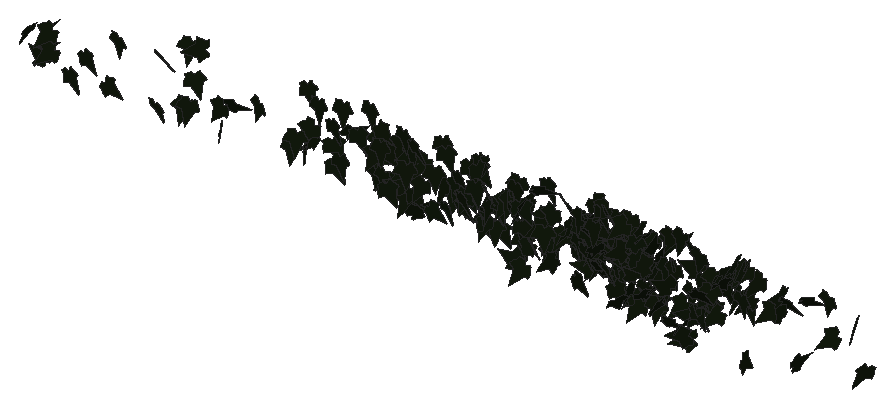
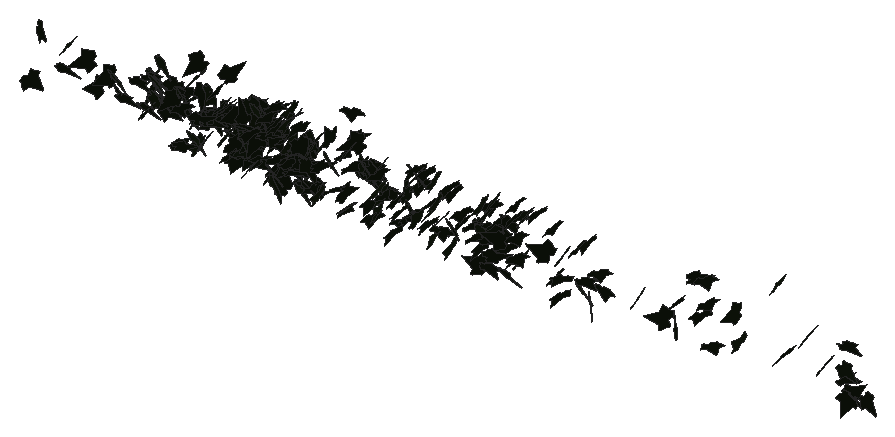
# SketchUp Ruby script. Lengths in inches.
U = 1.inch
M = Sketchup.active_model
def pt(a) = Geom::Point3d.new(a.map { |v| v * U })
def face(e, loops, mat)
  f = e.add_face(loops[0].map { |a| pt(a) })
  loops[1..].each { |l| e.add_face(l.map { |a| pt(a) }).erase! }
  f.material = f.back_material = mat if mat
  f
end
# faces: each face lists its corners as indices into pts; further lists are holes
def faces(e, pts, list, mat = nil) = list.each { |f| face(e, (f[0].is_a?(Array) ? f : [f]).map { |l| l.map { |i| pts[i] } }, mat) }
# xy, xz, yz: faces in a plane at the given z, y or x. An outline is a flat list of corners, or four numbers for a rectangle; further outlines are holes
def ring(l) = l.size == 4 ? [[l[0], l[1]], [l[2], l[1]], [l[2], l[3]], [l[0], l[3]]] : l.each_slice(2).to_a
def flat(e, list, mat, &to3) = list.each { |f| face(e, (f[0].is_a?(Array) ? f : [f]).map { |l| ring(l).map { |u, v| to3.(u, v) } }, mat) }
def xy(e, z, list, mat = nil) = flat(e, list, mat) { |x, y| [x, y, z] }
def xz(e, y, list, mat = nil) = flat(e, list, mat) { |x, z| [x, y, z] }
def yz(e, x, list, mat = nil) = flat(e, list, mat) { |y, z| [x, y, z] }
def lines(e, pts, list) = list.each { |a, b| e.add_line(pt(pts[a]), pt(pts[b])) }
# prism: a flat outline (further loops are holes) pulled along v
def prism(e, loops, v, mat = nil)
  f = face(e, loops, mat); d = Geom::Vector3d.new(v.map { |x| x * U })
  f.pushpull(f.normal.samedirection?(d) ? d.length : -d.length)
end
def box(e, o, s, mat = nil) = prism(e, [[o, [o[0] + s[0], o[1], o[2]], [o[0] + s[0], o[1] + s[1], o[2]], [o[0], o[1] + s[1], o[2]]]], [0, 0, s[2]], mat)
def at(x, y, z, deg = 0) = Geom::Transformation.translation(pt([x, y, z])) * Geom::Transformation.rotation(ORIGIN, Z_AXIS, deg.degrees)
def axes(o, x, y, z) = Geom::Transformation.new([*x, 0, *y, 0, *z, 0, *pt(o).to_a, 1])
def part(name) = M.definitions.add(name)
# library, detail: a bought-in or finely detailed component or shape, given as its bounding box
def library(name, o, s) = part(name).tap { |d| box(d.entities, o, s) }
def detail(e, o, s) = box(e.add_group.entities, o, s)
def put(e, d, t, mat = nil) = e.add_instance(d, t).tap { |i| i.material = mat if mat }
def group(e, t, mat = nil) = e.add_group.tap { |g| g.transformation = t; g.material = mat if mat }.entities
root = M.entities
M.materials.add("efeu1").color = [18, 25, 13]
c1 = part("ivyleaf_9")
p = [[1.54,2.16,1.25],[1.36,2.04,1.19],[-0.21,0.99,0.68],[-0.71,1.11,0.82],[-0.85,0.86,0.67],[-0.8,0.17,0.21],
  [-0.9,-0.01,0.1],[-0.67,-0.16,-0.02],[-0.08,-0.08,-0.05],[-0.03,-0.6,-0.4],[0.65,-0.88,-0.66],[0.83,-0.6,-0.49],
  [1.29,-0.42,-0.43],[1.8125,-0.07,-0.26],[1.21,0.44,0.15]]
faces(c1.entities,p,[[0,1,2,3,4,5,6,7,8,9,10,11,12,13,14]],"efeu1")
put(root,c1,axes([46.6,216.37,258.25],[-0.27202,-0.34629,-0.23682],[0.19921,0.14178,-0.43614],[0.36922,-0.33163,0.06083]))
put(root,c1,axes([55.82,216.69,257.36],[0.0222,0.00311,0.4995],[-0.43747,-0.24121,0.02095],[0.2411,-0.43796,-0.00798]))
put(root,c1,axes([44.75,216.71,254.99],[-0.44174,-0.23377,0.01468],[-0.01267,-0.00744,-0.49978],[0.23389,-0.44192,0.00065]))
put(root,c1,axes([51.99,216.38,255.35],[0.13956,0.47976,-0.01875],[-0.00594,-0.0178,-0.49965],[-0.48009,0.13969,0.00073]))
put(root,c1,axes([57.05,216.84,254.52],[-0.16748,-0.06607,-0.46646],[-0.30465,-0.36244,0.16072],[-0.35936,0.33804,0.08114]))
put(root,c1,axes([57.76,216.6,257.77],[0.46943,0.14872,0.08669],[0.08408,0.02166,-0.4924],[-0.15022,0.47688,-0.00467]))
put(root,c1,axes([50.58,216.97,257.02],[0.32423,-0.35893,0.12668],[0.07945,-0.09892,-0.48364],[0.37224,0.33374,-0.00711]))
put(root,c1,axes([61.5,216.62,254.54],[0.14205,-0.0765,-0.47325],[-0.35114,0.31944,-0.15703],[0.32638,0.37697,0.03702]))
put(root,c1,axes([57.02,217.34,253.99],[-0.31084,-0.10965,0.37597],[-0.32126,-0.20314,-0.32485],[0.22399,-0.44352,0.05583]))
put(root,c1,axes([56.46,217.125,254.9],[-0.19577,0.41436,-0.19996],[0.08916,-0.17901,-0.45826],[-0.45136,-0.21508,-0.0038]))
put(root,c1,axes([55.3125,216.99,254.87],[0.44843,-0.00718,0.22104],[0.22112,0.02369,-0.44782],[-0.00405,0.49939,0.02442]))
put(root,c1,axes([45.39,217.83,257.31],[-0.21869,-0.24197,0.37898],[-0.22849,-0.30316,-0.3254],[0.38726,-0.31551,0.02202]))
put(root,c1,axes([43.55,217.49,254.54],[-0.15058,0.15267,0.45168],[-0.42718,0.16718,-0.19892],[-0.21176,-0.4458,0.08009]))
put(root,c1,axes([12.92,217.94,258.77],[0.08923,-0.44015,0.21978],[0.07683,-0.20816,-0.44807],[0.48594,0.11373,0.03048]))
put(root,c1,axes([44.5,217.96,255.54],[-0.00907,-0.19475,0.46042],[0.18666,-0.42852,-0.17758],[0.46376,0.16867,0.08047]))
put(root,c1,axes([50.88,217.7,255.39],[0.15521,-0.37076,-0.2974],[-0.03273,0.30378,-0.39579],[0.47417,0.14233,0.07003]))
put(root,c1,axes([56.61,218.16,255.05],[-0.21741,0.01252,0.45009],[-0.3715,-0.28738,-0.17145],[0.2544,-0.40897,0.13426]))
put(root,c1,axes([51.73,218.16,255.46],[-0.16544,0.16469,-0.44216],[0.31866,-0.30655,-0.23341],[-0.34797,-0.35903,-0.00352]))
put(root,c1,axes([53.93,217.61,254.95],[0.08311,0.39802,0.29098],[0.07803,0.28075,-0.40631],[-0.48683,0.11295,-0.01545]))
put(root,c1,axes([51.03,218.4,257.45],[-0.17348,-0.17204,0.43624],[-0.29823,-0.31848,-0.24419],[0.36189,-0.34492,0.00789]))
put(root,c1,axes([52.95,218.23,257.14],[-0.34233,0.00365,0.36441],[-0.36442,0.00068,-0.34234],[-0.00299,-0.49999,0.0022]))
put(root,c1,axes([44,218.26,255.5],[-0.49518,-0.06094,-0.03293],[0.0327,0.00393,-0.49891],[0.06106,-0.49626,0.00009]))
put(root,c1,axes([55.6875,218.3,255.66],[-0.48249,-0.12906,0.02348],[-0.02308,-0.00461,-0.49945],[0.12913,-0.48303,-0.00151]))
put(root,c1,axes([8.98,218.17,255],[0.23883,-0.4254,-0.10953],[-0.03464,0.10604,-0.4874],[0.43791,0.2404,0.02117]))
put(root,c1,axes([18,218.39,256],[-0.17042,-0.46998,-0.00871],[-0.00292,0.01032,-0.49988],[0.47005,-0.17033,-0.00627]))
put(root,c1,axes([38.69,218.25,257.01],[0.3155,-0.38699,0.02646],[0.01015,-0.02586,-0.49923],[0.38776,0.31555,-0.00846]))
put(root,c1,axes([10.19,218.15,256.64],[0.27225,-0.38072,-0.17588],[-0.05784,0.1736,-0.46531],[0.41537,0.27371,0.05048]))
put(root,c1,axes([52.14,218.26,257.62],[0.07993,-0.37701,-0.31856],[-0.0011,0.32257,-0.38203],[0.49357,0.06177,0.05074]))
put(root,c1,axes([7.3,218.61,257.05],[-0.45431,-0.19542,0.07356],[-0.07134,-0.02028,-0.49447],[0.19624,-0.45978,-0.00946]))
put(root,c1,axes([56.44,218.5,255.39],[0.18945,-0.43156,-0.16691],[-0.06005,0.15591,-0.47126],[0.45881,0.19861,0.00725]))
put(root,c1,axes([51.76,218.54,255.93],[0.06218,0.09947,0.48604],[-0.49051,0.08578,0.0452],[-0.07439,-0.48244,0.10825]))
put(root,c1,axes([64.18,218.15,254.37],[0.07503,0.11513,0.48074],[0.29064,0.38305,-0.1371],[-0.39987,0.30002,-0.00944]))
put(root,c1,axes([34.2,218.72,257.2],[-0.16152,-0.45144,-0.14182],[0.04335,0.13511,-0.47944],[0.4712,-0.16717,-0.0045]))
put(root,c1,axes([36.31,218.41,255.3],[0.2751,-0.28143,-0.3084],[-0.09944,0.31454,-0.37574],[0.4055,0.26807,0.11709]))
put(root,c1,axes([31.8,218.94,257.28],[-0.20715,-0.42551,0.16133],[-0.03674,-0.16104,-0.47193],[0.45359,-0.20737,0.03545]))
put(root,c1,axes([32.16,218.84,257.95],[0.01535,-0.49936,0.02005],[0.00157,-0.02001,-0.4996],[0.49976,0.0154,0.00095]))
put(root,c1,axes([11.61,218.45,255.0625],[0.28954,-0.28549,-0.29097],[-0.07063,0.31636,-0.38069],[0.40147,0.26155,0.14287]))
put(root,c1,axes([59.54,218.91,257.1],[0.1146,-0.46397,0.14697],[0.06046,-0.13625,-0.47726],[0.48292,0.12716,0.02488]))
put(root,c1,axes([51.8,218.98,253.98],[-0.35344,-0.34688,0.06897],[-0.0423,-0.05534,-0.49512],[0.35113,-0.35583,0.00977]))
put(root,c1,axes([48.54,218.79,255.3],[0.24621,-0.18445,0.39415],[0.33599,-0.20724,-0.30686],[0.27657,0.41597,0.0219]))
put(root,c1,axes([51.61,218.85,258.23],[-0.29685,-0.24752,-0.3172],[0.30386,0.12045,-0.37836],[0.26372,-0.4174,0.07891]))
put(root,c1,axes([57.3,218.85,256.98],[-0.29515,-0.33546,-0.22439],[0.16685,0.15171,-0.44626],[0.36749,-0.33831,0.02238]))
put(root,c1,axes([57,219.11,256.3],[-0.2397,-0.33909,0.2785],[-0.02799,-0.30488,-0.3953],[0.43791,-0.2051,0.12717]))
put(root,c1,axes([14.9375,218.95,254.57],[0.20312,-0.40476,0.21192],[0.14685,-0.16178,-0.44974],[0.43264,0.24494,0.05315]))
put(root,c1,axes([46.95,218.88,254.0625],[-0.00252,-0.04185,-0.49824],[0.4782,0.14529,-0.01462],[0.146,-0.47659,0.0393]))
put(root,c1,axes([44.99,219.23,254.45],[0.00054,-0.18494,-0.46454],[0.18893,-0.43002,0.17142],[-0.46293,-0.17572,0.06942]))
put(root,c1,axes([30.33,218.94,258.12],[0.10182,-0.46175,-0.16255],[0.03884,0.17312,-0.46746],[0.48798,0.08256,0.07112]))
put(root,c1,axes([46.87,219.21,256.47],[0.13455,-0.44972,0.17217],[0.05309,-0.16382,-0.46941],[0.47862,0.1446,0.00366]))
put(root,c1,axes([51.33,218.93,254.42],[0.02387,-0.38738,-0.31522],[0.11928,0.31087,-0.373],[0.48498,-0.05739,0.10725]))
put(root,c1,axes([48.82,219.1,255.74],[-0.4367,0.13125,-0.2051],[0.18228,-0.10302,-0.45405],[-0.16145,-0.47134,0.04213]))
put(root,c1,axes([53.73,219.13,257.28],[-0.37507,-0.11711,-0.3092],[0.29288,0.09933,-0.39288],[0.15345,-0.47584,-0.00592]))
put(root,c1,axes([52.93,219.24,254.33],[-0.14871,-0.47622,-0.03324],[0.00979,0.03176,-0.49889],[0.47727,-0.14903,-0.00012]))
put(root,c1,axes([50.2,219.23,257.27],[0.0615,-0.49608,0.01088],[-0.00534,-0.01163,-0.49984],[0.49617,0.06136,-0.00673]))
put(root,c1,axes([54.16,219.37,257.08],[-0.03919,-0.46359,0.18317],[0.0017,-0.18386,-0.46497],[0.49846,-0.03582,0.01599]))
put(root,c1,axes([32.47,219.05,255.14],[0.07068,-0.42142,-0.25964],[0.01915,0.26441,-0.42394],[0.49461,0.04999,0.05352]))
put(root,c1,axes([6.82,219.39,255.21],[-0.3187,-0.30322,0.23768],[-0.17883,-0.15679,-0.43981],[0.34125,-0.36534,-0.00851]))
put(root,c1,axes([38.01,219.03,255.89],[0.34804,-0.30238,-0.19348],[-0.09375,0.18356,-0.45554],[0.34652,0.35337,0.07108]))
put(root,c1,axes([51.11,219.29,256.08],[-0.23991,0.03835,0.437],[-0.43764,-0.05521,-0.23542],[0.0302,-0.49546,0.06006]))
put(root,c1,axes([19.54,219.53,255.84],[-0.13919,-0.38832,0.28255],[-0.02579,-0.28771,-0.40812],[0.47954,-0.12818,0.06006]))
put(root,c1,axes([51.93,218.82,254.7],[0.27637,0.4073,0.08789],[0.04051,0.0787,-0.4921],[-0.4147,0.27912,0.0105]))
put(root,c1,axes([50.17,219.55,258.52],[-0.28732,-0.33465,0.2355],[-0.12388,-0.20312,-0.43977],[0.39,-0.31105,0.03381]))
put(root,c1,axes([55.93,219.54,258.43],[-0.02564,-0.44129,0.23367],[0.07628,-0.2347,-0.43486],[0.49348,0.01335,0.07936]))
put(root,c1,axes([38.08,219.5625,256.24],[-0.14057,-0.44203,0.18669],[0.02208,-0.20028,-0.4576],[0.47933,-0.1204,0.07582]))
put(root,c1,axes([25.34,219.4,255.98],[-0.23511,-0.41805,-0.14128],[0.11602,0.09588,-0.47681],[0.42575,-0.25699,0.05191]))
put(root,c1,axes([47.24,219.42,255.93],[0.19824,-0.44635,0.10709],[0.04649,-0.09653,-0.48839],[0.45666,0.20359,0.00323]))
put(root,c1,axes([6.26,219.26,254.35],[0.05843,0.08654,0.43977],[-0.46088,0.07463,0.0409],[-0.0699,-0.41972,0.09794]))
put(root,c1,axes([19.44,219.41,253.81],[-0.0579,0.27116,0.41608],[0.00919,-0.41824,0.27385],[0.49655,0.03937,0.04345]))
put(root,c1,axes([51.8,219.36,258.32],[-0.25272,0.35464,-0.24569],[0.01565,-0.27701,-0.41595],[-0.43115,-0.21793,0.12892]))
put(root,c1,axes([42.44,219.27,257.32],[-0.11561,-0.25294,-0.41552],[0.26195,0.32751,-0.27225],[0.4099,-0.28064,0.05679]))
put(root,c1,axes([50.92,219.54,256.4],[-0.42153,-0.11595,-0.24263],[0.25964,-0.05806,-0.42334],[0.07,-0.48289,0.10916]))
put(root,c1,axes([57.39,219.28,257],[-0.37985,0.32233,0.04262],[-0.03893,0.01998,-0.49808],[-0.3228,-0.38171,0.00992]))
put(root,c1,axes([38.875,219.47,257.24],[-0.01632,-0.48334,-0.12694],[-0.00554,0.12718,-0.48352],[0.4997,-0.01437,-0.00951]))
put(root,c1,axes([57.7,219.07,257.33],[0.1816,0.46233,0.05721],[0.029,0.05007,-0.49664],[-0.46495,0.18369,-0.00863]))
put(root,c1,axes([58.875,219.55,256.9],[-0.4172,0.05536,-0.26996],[0.26086,-0.07858,-0.41926],[-0.08885,-0.49067,0.03668]))
put(root,c1,axes([48.04,219.52,256.23],[-0.08518,0.30537,-0.38664],[0.08176,-0.37818,-0.3167],[-0.48586,-0.11718,0.01449]))
put(root,c1,axes([44.61,219.75,257.34],[-0.14301,-0.44657,0.17356],[-0.03051,-0.17227,-0.46839],[0.47814,-0.14456,0.02203]))
put(root,c1,axes([39.48,219.71,255.04],[-0.14928,-0.46948,0.08546],[-0.0198,-0.08338,-0.4926],[0.47678,-0.15045,0.0063]))
put(root,c1,axes([42.54,219.63,257.2],[-0.20433,0.20114,-0.40962],[0.19872,-0.36481,-0.27826],[-0.41081,-0.27651,0.06914]))
put(root,c1,axes([24.83,219.67,255.18],[-0.36365,-0.22218,-0.26152],[0.24509,0.09856,-0.42452],[0.24019,-0.43694,0.03723]))
put(root,c1,axes([43.96,219.85,256.8125],[-0.19323,-0.44485,0.12152],[-0.03486,-0.11729,-0.4848],[0.45983,-0.19583,0.01431]))
put(root,c1,axes([58.67,219.51,258.83],[-0.35517,0.34586,-0.06512],[0.04753,-0.04453,-0.49574],[-0.34871,-0.35833,-0.00124]))
put(root,c1,axes([47.68,219.8,257.49],[-0.01573,-0.4963,0.05865],[-0.00361,-0.05856,-0.49655],[0.49974,-0.01605,-0.00174]))
put(root,c1,axes([67.64,219.72,257.95],[-0.24893,0.16868,-0.39947],[0.34126,-0.20799,-0.30048],[-0.26754,-0.42224,-0.01157]))
put(root,c1,axes([31.91,219.58,257.21],[-0.04556,-0.19176,-0.45952],[0.40278,0.25709,-0.14722],[0.29274,-0.38358,0.13105]))
put(root,c1,axes([47.2,219.74,256.875],[0.09362,-0.49074,-0.02032],[-0.00635,0.01947,-0.49958],[0.49112,0.0938,-0.00259]))
put(root,c1,axes([51.35,219.27,256.04],[0.39024,0.27499,0.14864],[0.12242,0.08432,-0.47739],[-0.28763,0.40898,-0.00152]))
put(root,c1,axes([49.41,219.95,254.32],[-0.06597,-0.38801,0.30838],[0.08309,-0.31536,-0.37901],[0.48862,0.00124,0.10608]))
put(root,c1,axes([46.54,219.96,257.63],[-0.03361,-0.4324,0.24879],[0.01186,-0.24998,-0.43286],[0.49873,-0.0232,0.02706]))
put(root,c1,axes([45.82,219.69,256.78],[-0.43317,0.19042,-0.16156],[0.14963,-0.06106,-0.47316],[-0.19993,-0.45827,-0.00409]))
put(root,c1,axes([46.97,219.52,256.74],[0.34698,-0.06127,0.35475],[0.35388,-0.03248,-0.35173],[0.06615,0.49517,0.02082]))
put(root,c1,axes([48.15,219.74,258.73],[0.21227,-0.45054,-0.04421],[-0.01463,0.04198,-0.49802],[0.45247,0.21273,0.00464]))
put(root,c1,axes([38.26,219.67,258.42],[0.05787,-0.45014,-0.20982],[-0.02566,0.20825,-0.45384],[0.49598,0.06329,0.00101]))
put(root,c1,axes([39.46,219.65,255],[0.11746,-0.43417,-0.2184],[0.01219,0.22724,-0.44521],[0.48585,0.09927,0.06397]))
put(root,c1,axes([45.36,219.93,258.125],[0.04871,-0.28251,0.40965],[0.23061,-0.35193,-0.27012],[0.44096,0.21525,0.09601]))
put(root,c1,axes([55.43,219.78,254.25],[0.32276,-0.34337,0.16709],[0.12139,-0.11518,-0.47117],[0.36206,0.34472,0.00901]))
put(root,c1,axes([38.92,219.62,258.45],[0.1207,-0.39132,-0.28688],[0.02892,0.3009,-0.39828],[0.48435,0.07955,0.09527]))
put(root,c1,axes([30.82,220,255.07],[0.06163,-0.43045,0.24682],[0.07195,-0.23833,-0.43361],[0.49094,0.08896,0.03257]))
put(root,c1,axes([51.9375,219.64,257.16],[0.15074,0.43426,0.19672],[-0.14434,-0.15506,0.4529],[0.45436,-0.19332,0.07861]))
put(root,c1,axes([51,219.57,257.68],[0.47929,-0.07838,-0.1189],[-0.11557,0.02987,-0.48554],[0.08322,0.49291,0.01051]))
put(root,c1,axes([43.39,219.4375,258.5],[0.40839,0.07632,0.2782],[0.25013,0.14655,-0.40738],[-0.14372,0.47191,0.08152]))
put(root,c1,axes([49.49,219.89,254.8],[-0.00975,-0.49227,-0.08706],[-0.00631,0.08719,-0.4923],[0.49987,-0.0085,-0.00791]))
put(root,c1,axes([52.46,219.3,254.99],[0.18266,0.30273,0.35354],[0.07102,0.35721,-0.34257],[-0.45999,0.17537,0.08749]))
put(root,c1,axes([39.45,220.05,256.4],[-0.11054,-0.16565,0.45863],[0.19002,-0.44772,-0.11592],[0.44908,0.14867,0.16193]))
put(root,c1,axes([48.29,220.17,258.7],[-0.27907,-0.32527,0.25752],[0.00219,-0.31151,-0.3911],[0.41486,-0.21716,0.17529]))
put(root,c1,axes([47.47,219.94,254.36],[-0.27255,0.08941,0.40954],[-0.41415,-0.13295,-0.24659],[0.0648,-0.47363,0.14653]))
put(root,c1,axes([39.5625,219.91,256.1],[-0.37761,0.02738,-0.32659],[0.32594,-0.02066,-0.3786],[-0.03423,-0.49882,-0.00225]))
put(root,c1,axes([52.46,219.84,254.27],[-0.1332,-0.38103,-0.29508],[0.14755,0.2592,-0.40131],[0.45879,-0.19399,0.04339]))
put(root,c1,axes([47.04,219.39,257.375],[0.00163,0.32837,0.37706],[-0.00542,0.37705,-0.32833],[-0.49997,-0.00302,0.00479]))
put(root,c1,axes([35.37,219.97,256.82],[-0.08758,-0.47914,-0.11291],[0.02117,0.11092,-0.48708],[0.49181,-0.0901,0.00085]))
put(root,c1,axes([34.3125,220.16,255.52],[-0.20038,-0.43686,0.13785],[-0.02232,-0.14098,-0.47919],[0.45755,-0.1982,0.037]))
put(root,c1,axes([42.77,219.94,257.33],[-0.45332,0.11996,-0.17352],[0.1712,-0.03107,-0.46875],[-0.12324,-0.4844,-0.01291]))
put(root,c1,axes([33.89,219.76,255.01],[0.15219,-0.36221,-0.30926],[-0.07521,0.30232,-0.39109],[0.4703,0.16555,0.03754]))
put(root,c1,axes([39.85,220.06,254.73],[-0.13594,-0.47028,-0.10176],[0.12337,0.06814,-0.47973],[0.46508,-0.15554,0.09751]))
put(root,c1,axes([41.4,220.08,257.84],[0.13605,-0.47249,0.09079],[0.0135,-0.09056,-0.49154],[0.48095,0.1362,-0.01189]))
put(root,c1,axes([65.77,220.04,256.08],[-0.47969,-0.05259,0.13088],[-0.12898,-0.02426,-0.48247],[0.05709,-0.49663,0.00971]))
put(root,c1,axes([49.54,219.9375,257.04],[-0.17822,0.36622,-0.29003],[0.10549,-0.27085,-0.40683],[-0.45509,-0.2062,0.01928]))
put(root,c1,axes([51.18,219.82,258.29],[-0.36322,0.3421,0.03215],[-0.0245,0.02087,-0.49896],[-0.34274,-0.36405,0.0016]))
put(root,c1,axes([28.09,220.08,255.02],[0.10217,-0.48944,0.00234],[-0.00588,-0.00362,-0.49995],[0.48941,0.10214,-0.00649]))
put(root,c1,axes([33.97,219.68,253.45],[0.03939,-0.07263,0.49313],[0.46988,0.17045,-0.01242],[-0.1663,0.4644,0.08169]))
put(root,c1,axes([48.58,220.11,257.24],[0.01199,-0.49917,-0.02615],[0.10814,0.02813,-0.48735],[0.48802,0.00603,0.10864]))
put(root,c1,axes([6.29,219.98,256.51],[-0.23745,0.30854,-0.2223],[0.0147,-0.241,-0.37636],[-0.40511,-0.1896,0.11664]))
put(root,c1,axes([32.82,220.16,258.38],[0.14645,-0.45808,0.13682],[0.04076,-0.13061,-0.48092],[0.47633,0.15202,-0.00091]))
put(root,c1,axes([52.05,219.69,255.99],[-0.2006,0.43442,0.14504],[-0.05858,0.1327,-0.4785],[-0.45423,-0.20896,-0.00235]))
put(root,c1,axes([58.75,220.03,256.48],[-0.3536,0.26334,-0.23583],[0.14283,-0.1987,-0.43602],[-0.32337,-0.37573,0.0653]))
put(root,c1,axes([5.47,220.13,254.77],[-0.39607,-0.10088,-0.21953],[0.24396,-0.05052,-0.38304],[0.06577,-0.42012,0.09877]))
put(root,c1,axes([68.05,220.16,254.67],[-0.02731,0.194,-0.46002],[0.09766,-0.44973,-0.19545],[-0.48961,-0.10052,-0.01333]))
put(root,c1,axes([17.61,220.25,258.62],[-0.26901,-0.10497,0.40819],[-0.35325,-0.20798,-0.28629],[0.22989,-0.44241,0.03774]))
put(root,c1,axes([52.91,220.07,256.0625],[-0.4974,0.04997,0.00987],[-0.01011,-0.00187,-0.49989],[-0.04993,-0.49749,0.00287]))
put(root,c1,axes([39.18,219.97,258.47],[-0.44,0.23485,0.0353],[-0.03332,0.01254,-0.49873],[-0.23514,-0.44124,0.00462]))
put(root,c1,axes([16.72,220.17,258.88],[-0.25462,-0.42066,-0.09064],[0.044,0.07931,-0.4917],[0.42806,-0.25837,-0.00337]))
put(root,c1,axes([36.99,220.03,257.02],[0.32808,-0.3769,-0.01767],[-0.01034,0.01443,-0.49968],[0.37717,0.32824,0.00168]))
put(root,c1,axes([58.6875,220.02,258.1],[-0.44814,0.21718,-0.0448],[0.03483,-0.03083,-0.49783],[-0.219,-0.44931,0.0125]))
put(root,c1,axes([14.31,219.95,257.35],[0.45402,-0.19269,0.08207],[0.07372,-0.03636,-0.4932],[0.19604,0.45994,-0.00461]))
put(root,c1,axes([52.65,219.57,257.13],[0.1633,0.19798,0.42911],[0.20739,0.37793,-0.25329],[-0.42465,0.26071,0.04132]))
put(root,c1,axes([51.01,219.68,256.37],[0.27802,0.41223,0.05267],[0.02808,0.04459,-0.49722],[-0.41463,0.27943,0.00164]))
put(root,c1,axes([36.12,220.08,258.37],[0.07221,-0.47026,-0.15375],[0.02536,0.1587,-0.47347],[0.49411,0.06058,0.04677]))
put(root,c1,axes([16.24,220.24,254.59],[-0.31196,-0.38528,-0.0651],[0.06464,0.03127,-0.49482],[0.38536,-0.31714,0.0303]))
put(root,c1,axes([55.8,219.88,254.76],[-0.29382,0.37778,0.14475],[-0.1414,0.07172,-0.4742],[-0.37905,-0.31959,0.06469]))
put(root,c1,axes([43.92,220.38,254.05],[-0.15103,-0.42974,0.20619],[-0.02696,-0.20825,-0.45377],[0.47588,-0.14819,0.03973]))
put(root,c1,axes([31.23,220.32,254.99],[0.00938,-0.47262,0.16291],[0.02075,-0.16243,-0.47243],[0.49948,0.01563,0.01657]))
put(root,c1,axes([33.625,220.03,258],[0.3574,-0.34695,-0.04349],[-0.02009,0.04171,-0.49785],[0.34909,0.35761,0.01588]))
put(root,c1,axes([48.23,219.83,255.7],[0.48837,0.10459,0.02364],[0.02243,0.00813,-0.49943],[-0.10486,0.48887,0.00325]))
put(root,c1,axes([47.67,220.04,254.44],[-0.36225,0.33955,-0.05899],[0.03745,-0.0463,-0.49644],[-0.3426,-0.36409,0.00811]))
put(root,c1,axes([38.41,220.39,255.26],[0.08257,-0.33871,0.35841],[0.17649,-0.31903,-0.34215],[0.46047,0.18301,0.06687]))
put(root,c1,axes([51.09,220.37,254.39],[0.08919,-0.46897,0.14871],[0.0506,-0.14158,-0.47686],[0.48937,0.10011,0.02221]))
put(root,c1,axes([33.15,220.29,254.1],[-0.45262,-0.19186,-0.09125],[0.08021,0.04455,-0.49151],[0.19673,-0.45957,-0.00955]))
put(root,c1,axes([47.66,220.11,257.28],[0.19061,-0.4113,-0.21094],[-0.05497,0.20638,-0.45209],[0.45896,0.19554,0.03346]))
put(root,c1,axes([41.04,220.03,256.26],[0.40959,-0.23557,-0.16355],[-0.13388,0.0951,-0.47226],[0.2536,0.43066,0.01483]))
put(root,c1,axes([46.73,220.31,255.27],[0.1796,-0.46496,0.03948],[0.00829,-0.03912,-0.4984],[0.46656,0.17968,-0.00634]))
put(root,c1,axes([53.79,220.46,258.64],[-0.01471,-0.46051,0.19419],[-0.00366,-0.19417,-0.46074],[0.49977,-0.01498,0.00235]))
put(root,c1,axes([46.02,220.5,256.28],[-0.25798,-0.1737,0.3915],[-0.27847,-0.27923,-0.30739],[0.32543,-0.37664,0.04733]))
put(root,c1,axes([40.04,220.31,256.16],[0.08128,-0.49248,-0.02921],[0.00102,0.02977,-0.49911],[0.49335,0.08107,0.00584]))
put(root,c1,axes([48.25,220.26,258.47],[0.32211,-0.3709,0.09316],[0.05087,-0.07917,-0.49106],[0.37902,0.32584,-0.01327]))
put(root,c1,axes([35.96,220.28,255.92],[-0.43804,0.05766,-0.23408],[0.23249,-0.0274,-0.44181],[-0.06378,-0.49591,-0.00281]))
put(root,c1,axes([28.08,220.4,258.49],[-0.00123,-0.4997,0.01739],[-0.00128,-0.01738,-0.4997],[0.5,-0.00128,-0.00124]))
put(root,c1,axes([48.36,220.47,255.76],[-0.36789,-0.1714,0.29203],[-0.25007,-0.15322,-0.40496],[0.22831,-0.44401,0.02701]))
put(root,c1,axes([54.96,220.01,258.42],[0.31998,0.11374,-0.36698],[-0.36446,-0.06129,-0.33677],[-0.12159,0.48302,0.04369]))
put(root,c1,axes([32.9375,220.36,254.78],[-0.22828,0.01631,0.44455],[-0.44081,-0.07547,-0.22359],[0.0598,-0.494,0.04883]))
put(root,c1,axes([40.6,220.45,256.52],[-0.39095,-0.31159,-0.00842],[0.02803,-0.02168,-0.49874],[0.31045,-0.39043,0.03442]))
put(root,c1,axes([33.9,220.16,256.7],[-0.32457,0.36664,-0.10114],[0.07012,-0.073,-0.48965],[-0.37381,-0.33204,-0.00403]))
put(root,c1,axes([58.8,220.1875,258.19],[-0.39153,0.3052,-0.05963],[0.04402,-0.04051,-0.49641],[-0.30784,-0.39397,0.00486]))
put(root,c1,axes([41.82,220.32,254.45],[-0.07029,-0.46452,-0.17112],[0.03179,0.16825,-0.46977],[0.49401,-0.07691,0.00588]))
put(root,c1,axes([61.76,219.93,256.125],[-0.11586,0.20755,0.43989],[-0.22942,0.37541,-0.23755],[-0.42888,-0.25689,0.00824]))
put(root,c1,axes([57.67,220.23,256.26],[-0.11562,0.11941,-0.47157],[-0.39518,-0.3057,0.01948],[-0.28367,0.37721,0.16506]))
put(root,c1,axes([41.32,220.51,254.79],[0.12533,-0.35813,0.32563],[0.11487,-0.30475,-0.37938],[0.47021,0.1699,0.00589]))
put(root,c1,axes([58.75,220.47,258.12],[-0.43464,-0.24577,0.0263],[-0.01177,-0.03256,-0.4988],[0.24689,-0.43421,0.02252]))
put(root,c1,axes([16.83,220.3125,256.55],[-0.03033,-0.45532,-0.20436],[0.07811,0.19788,-0.45248],[0.49293,-0.05938,0.05913]))
put(root,c1,axes([56.54,220.54,254.28],[-0.34848,-0.30645,0.18615],[-0.14324,-0.11899,-0.46403],[0.3287,-0.37674,-0.00486]))
put(root,c1,axes([33.25,220.47,257.48],[0.0591,-0.49158,0.06972],[-0.00287,-0.07055,-0.49499],[0.49649,0.05811,-0.01116]))
put(root,c1,axes([49.85,220.52,258.44],[-0.15241,-0.47326,0.05286],[0.00411,-0.05681,-0.49675],[0.47619,-0.15099,0.0212]))
put(root,c1,axes([33.15,220.52,256.01],[-0.40656,-0.22385,0.186],[-0.16095,-0.0933,-0.4641],[0.24249,-0.43725,0.00381]))
put(root,c1,axes([41.84,220.27,255.39],[-0.00652,-0.42293,-0.26662],[0.05466,0.26444,-0.42081],[0.49696,-0.03463,0.04279]))
put(root,c1,axes([49.25,220.08,255.16],[0.25168,-0.26523,-0.34104],[-0.16355,0.30683,-0.35932],[0.39989,0.29242,0.06769]))
put(root,c1,axes([31.02,220.15,258.16],[0.24717,-0.3425,-0.26759],[-0.05633,0.27999,-0.4104],[0.43097,0.23303,0.09982]))
put(root,c1,axes([52.32,220.62,255.82],[-0.07972,-0.06969,-0.48866],[0.07923,-0.49038,0.05701],[-0.4872,-0.06835,0.08923]))
put(root,c1,axes([48.5,220.23,253.96],[0.10197,-0.0913,0.4809],[0.46981,-0.11964,-0.12234],[0.13741,0.47681,0.06139]))
put(root,c1,axes([35.71,220.43,254.4],[0.27338,-0.40005,0.12337],[0.06531,-0.10479,-0.48451],[0.41352,0.28103,-0.00504]))
put(root,c1,axes([48.04,220.52,256.22],[-0.18302,-0.4646,-0.0255],[0.03368,0.01411,-0.49866],[0.46408,-0.18425,0.02613]))
put(root,c1,axes([41.27,220.23,256.45],[0.35089,-0.33417,-0.12334],[-0.02928,0.14548,-0.47747],[0.355,0.3423,0.08253]))
put(root,c1,axes([56.26,220.5,256.88],[-0.22654,-0.43876,-0.07856],[0.03611,0.06976,-0.49379],[0.44427,-0.2294,0.00008]))
put(root,c1,axes([54.43,220.59,255.09],[0.05892,-0.45218,0.20508],[0.02971,-0.20294,-0.456],[0.49563,0.06592,0.00295]))
put(root,c1,axes([36.55,220.65,256],[-0.06091,-0.42843,0.25048],[0.04791,-0.25626,-0.42666],[0.49396,-0.02797,0.07227]))
put(root,c1,axes([32.6,220.37,256.96],[-0.28955,-0.23416,-0.33366],[0.25342,0.21716,-0.37232],[0.31928,-0.38472,-0.00707]))
put(root,c1,axes([61.67,220.1875,257.01],[0.47503,-0.04904,0.14812],[0.14563,-0.03101,-0.47732],[0.056,0.49662,-0.01518]))
put(root,c1,axes([60.81,220.49,255.99],[-0.48155,-0.07535,0.1115],[-0.10849,-0.02779,-0.4873],[0.07963,-0.49351,0.01042]))
put(root,c1,axes([49.61,220.4,255.03],[-0.46355,0.16973,-0.07947],[0.07166,-0.03538,-0.49357],[-0.17317,-0.46898,0.00847]))
put(root,c1,axes([47,220.3,255.76],[0.07066,-0.05032,0.49242],[-0.42276,0.25258,0.08647],[-0.25745,-0.42857,-0.00685]))
put(root,c1,axes([55.76,220.13,256.04],[-0.09477,0.14751,0.46825],[-0.32526,0.33835,-0.17242],[-0.36773,-0.33728,0.03183]))
put(root,c1,axes([52.84,220.42,256.11],[0.19319,-0.45353,-0.0836],[-0.025,0.08021,-0.49289],[0.46049,0.19462,0.00831]))
put(root,c1,axes([27.18,220.42,256.9375],[0.25058,-0.43074,-0.04087],[-0.01686,0.03748,-0.49831],[0.43235,0.25111,0.00426]))
put(root,c1,axes([32.31,220.7,257.39],[-0.10583,-0.45054,0.18923],[-0.00505,-0.1926,-0.46139],[0.48865,-0.09957,0.03621]))
put(root,c1,axes([46.48,220.55,257.3],[0.2262,-0.42741,0.12709],[0.05894,-0.1126,-0.48358],[0.442,0.23375,-0.00056]))
put(root,c1,axes([26.05,220.61,257.89],[0.06229,-0.49194,0.06412],[-0.00209,-0.06489,-0.49577],[0.4961,0.06149,-0.01014]))
put(root,c1,axes([47.27,220.41,257.64],[-0.07241,0.37962,-0.31724],[-0.02489,-0.32301,-0.38085],[-0.4941,-0.03936,0.06567]))
put(root,c1,axes([52.47,220.65,254.99],[-0.04149,-0.49482,0.05855],[0.0059,-0.05924,-0.49644],[0.49824,-0.0405,0.01076]))
put(root,c1,axes([52.76,220.75,257.93],[-0.13792,-0.44624,0.17846],[0.0002,-0.18572,-0.46423],[0.4806,-0.12798,0.05141]))
put(root,c1,axes([58.73,220.55,255.8],[0.14212,-0.47912,-0.01573],[-0.00119,0.01605,-0.49974],[0.47938,0.14208,0.00342]))
put(root,c1,axes([45.66,220.56,254.6],[0.27018,-0.40625,0.10938],[0.06081,-0.09092,-0.48789],[0.4163,0.27694,0.00028]))
put(root,c1,axes([34.06,220.76,256.68],[-0.262,-0.39283,0.16445],[-0.0374,-0.17111,-0.46832],[0.42422,-0.2577,0.06028]))
put(root,c1,axes([59.625,220.6,257.6],[-0.47728,-0.14826,-0.0148],[0.01475,0.00243,-0.49978],[0.14827,-0.47751,0.00205]))
put(root,c1,axes([21.36,220.76,256.06],[0.04114,-0.40295,0.29315],[0.02606,-0.292,-0.40504],[0.49762,0.04861,-0.00302]))
put(root,c1,axes([64.71,220.74,258.05],[0.01556,-0.43567,0.24485],[0.07753,-0.2399,-0.43178],[0.49371,0.05141,0.06009]))
put(root,c1,axes([57.02,220.07,257.22],[-0.00047,0.00705,-0.49995],[-0.10869,0.48799,0.00698],[0.48804,0.10869,0.00107]))
put(root,c1,axes([4.17,220.48,255.35],[-0.16746,0.31861,-0.26242],[0.09912,-0.23564,-0.3681],[-0.42761,-0.17939,0.01744]))
put(root,c1,axes([38.34,220.47,258.47],[0.23688,-0.42536,-0.11385],[-0.02705,0.11498,-0.48585],[0.4395,0.23633,0.03146]))
put(root,c1,axes([44.625,220.8,255.38],[-0.29237,-0.38055,0.14035],[0.02441,-0.18921,-0.46217],[0.40487,-0.2634,0.12922]))
put(root,c1,axes([40.66,220.74,256.48],[-0.16704,-0.46489,0.07731],[-0.0139,-0.07713,-0.49382],[0.47107,-0.16713,0.01284]))
put(root,c1,axes([31.87,220.27,256.1875],[0.18134,-0.05639,0.46253],[0.46256,0.08162,-0.1714],[-0.05617,0.49006,0.08177]))
put(root,c1,axes([36.4375,220.61,255.58],[-0.34027,-0.30599,-0.20146],[0.15882,0.12456,-0.45745],[0.33014,-0.37531,0.01243]))
put(root,c1,axes([52.72,220.82,258.16],[-0.11534,-0.44002,0.20754],[0.03103,-0.21952,-0.44816],[0.48552,-0.09051,0.07794]))
put(root,c1,axes([56.3,220.66,254.22],[-0.30845,0.03274,0.39215],[-0.38344,-0.13707,-0.29015],[0.0885,-0.47973,0.10967]))
put(root,c1,axes([47.74,220.43,257.34],[0.4324,-0.24869,-0.03442],[-0.01765,0.03827,-0.49822],[0.25044,0.43207,0.02432]))
put(root,c1,axes([61.45,220.36,257.13],[-0.33453,0.33409,0.16269],[-0.1314,0.09841,-0.47228],[-0.34759,-0.35874,0.02196]))
put(root,c1,axes([43.58,220.87,254.46],[-0.22839,-0.37322,0.24197],[0.06873,-0.29835,-0.39531],[0.43945,-0.14731,0.18758]))
put(root,c1,axes([27.3,220.49,254.27],[0.09373,-0.42885,-0.23937],[0.04205,0.24981,-0.43108],[0.48933,0.06068,0.0829]))
put(root,c1,axes([51.44,220.79,257.45],[-0.44286,-0.23005,-0.03083],[0.0955,-0.12006,-0.47588],[0.21155,-0.42739,0.15028]))
put(root,c1,axes([25.48,220.74,255.99],[-0.41423,-0.27946,0.01781],[-0.01446,-0.01041,-0.49968],[0.27965,-0.41448,0.00054]))
put(root,c1,axes([47.23,220.32,254.88],[-0.2602,0.23961,0.35339],[-0.25144,0.24848,-0.35361],[-0.34507,-0.36173,-0.00882]))
put(root,c1,axes([58.98,220.66,256.09],[-0.49918,-0.02794,0.00631],[-0.00478,-0.02742,-0.49922],[0.02824,-0.49846,0.02711]))
put(root,c1,axes([49.25,220.29,254.1875],[-0.21432,0.44098,0.09799],[-0.03428,0.09227,-0.49022],[-0.45043,-0.21685,-0.00932]))
put(root,c1,axes([54.21,220.09,258.23],[0.06769,0.30688,0.3889],[-0.02794,0.39425,-0.30624],[-0.49461,0.01973,0.07052]))
put(root,c1,axes([47.1875,220.3125,258.77],[0.17203,-0.26244,-0.38927],[-0.03991,0.40491,-0.29062],[0.46778,0.13106,0.11836]))
put(root,c1,axes([48.88,220.67,258.21],[0.05944,-0.49515,-0.03595],[-0.00508,0.0356,-0.49871],[0.49643,0.05965,-0.0008]))
put(root,c1,axes([24.9,220.61,253.7],[-0.11039,0.26714,0.40798],[0.03104,-0.41361,0.27923],[0.48667,0.08698,0.07474]))
put(root,c1,axes([49.82,220.82,257.3],[-0.40368,-0.1002,0.27749],[-0.22228,-0.20595,-0.39772],[0.194,-0.44446,0.12173]))
put(root,c1,axes([39.47,220.59,255.75],[0.15269,-0.45917,-0.12591],[0.00578,0.134,-0.48167],[0.47608,0.14564,0.04623]))
put(root,c1,axes([5.55,220.25,254.74],[0.26123,0.35864,0.04765],[0.02639,0.03879,-0.44988],[-0.38958,0.24311,0.00148]))
put(root,c1,axes([57.93,220.58,257.13],[-0.46054,0.18914,-0.04616],[0.04119,-0.02119,-0.49785],[-0.19029,-0.46236,0.00394]))
put(root,c1,axes([30.65,220.77,257.14],[-0.19921,-0.45756,-0.03093],[0.00836,0.03009,-0.49902],[0.45853,-0.19934,-0.00434]))
put(root,c1,axes([63.19,220.29,257.51],[0.41447,0.04368,0.27623],[0.25892,0.12675,-0.40853],[-0.10571,0.48169,0.08245]))
put(root,c1,axes([48.91,220.82,256.08],[-0.26172,-0.4252,0.02654],[-0.01335,-0.02294,-0.49929],[0.42582,-0.26206,0.00065]))
put(root,c1,axes([41.125,220.81,257.76],[-0.13433,-0.48125,0.01895],[0.00096,-0.01994,-0.4996],[0.48162,-0.13418,0.00628]))
put(root,c1,axes([35.4,220.6875,258.53],[0.0372,-0.48781,-0.10324],[-0.01197,0.10262,-0.48921],[0.49847,0.03887,-0.00404]))
put(root,c1,axes([50.875,220.67,257.1],[-0.01679,-0.47373,-0.15905],[0.05473,0.15644,-0.47173],[0.49671,-0.03325,0.0466]))
put(root,c1,axes([47.61,220.87,255.65],[-0.39202,-0.29859,0.08464],[-0.01762,-0.11473,-0.48634],[0.30986,-0.38429,0.07943]))
put(root,c1,axes([37.27,220.58,255.74],[0.11868,-0.43865,-0.20856],[0.01541,0.21799,-0.44971],[0.48547,0.10032,0.06527]))
put(root,c1,axes([43.35,220.65,258.5],[0.21151,-0.44858,-0.06358],[-0.0126,0.06431,-0.49569],[0.45289,0.21128,0.0159]))
put(root,c1,axes([19.3,220.45,255.375],[0.32171,-0.07983,0.37434],[0.37833,-0.00785,-0.32681],[0.05805,0.49352,0.05536]))
put(root,c1,axes([25.14,220.66,258.69],[0.11805,-0.46768,-0.13167],[-0.02919,0.12844,-0.48234],[0.48499,0.12157,0.00302]))
put(root,c1,axes([46.83,220.26,256.12],[0.38401,0.18819,0.25908],[0.21528,0.14774,-0.42641],[-0.23705,0.43904,0.03244]))
put(root,c1,axes([29.79,220.8,258.81],[0.12018,-0.47938,0.07584],[0.01586,-0.07421,-0.49421],[0.48508,0.12119,-0.00263]))
put(root,c1,axes([36.7,220.85,254.89],[0.15663,-0.41061,0.23846],[0.08175,-0.22403,-0.43946],[0.46774,0.17665,-0.00305]))
put(root,c1,axes([25.89,220.63,255.41],[-0.44439,0.22399,-0.04842],[0.0382,-0.03174,-0.49753],[-0.22596,-0.44589,0.0111]))
put(root,c1,axes([54.94,220.7,256.51],[-0.15659,0.09695,0.46484],[-0.47428,-0.008,-0.1581],[-0.02322,-0.49044,0.09447]))
put(root,c1,axes([30.56,220.86,255.81],[-0.27701,-0.41531,-0.02792],[0.01326,0.02472,-0.49921],[0.41604,-0.27732,-0.00269]))
put(root,c1,axes([27.07,220.65,255.6],[-0.00288,-0.40525,-0.29286],[0.19213,0.26948,-0.37479],[0.46161,-0.11469,0.15416]))
put(root,c1,axes([46.57,220.54,256.56],[-0.15559,0.4555,-0.13532],[0.01263,-0.13838,-0.4803],[-0.47501,-0.15288,0.03155]))
put(root,c1,axes([46.04,220.89,255.15],[-0.12116,-0.48402,0.03225],[-0.00371,-0.03231,-0.49894],[0.48508,-0.12115,0.00424]))
put(root,c1,axes([39.88,220.625,254.25],[0.1287,-0.42504,-0.22972],[-0.03947,0.22769,-0.4434],[0.48154,0.13227,0.02505]))
put(root,c1,axes([28.375,220.45,256.56],[0.11329,-0.09432,0.47777],[0.47889,0.11071,-0.0917],[-0.08849,0.47838,0.11542]))
put(root,c1,axes([31.6,220.6875,254.38],[-0.46521,0.12202,0.13671],[-0.13228,0.03448,-0.48095],[-0.1268,-0.48365,0.0002]))
